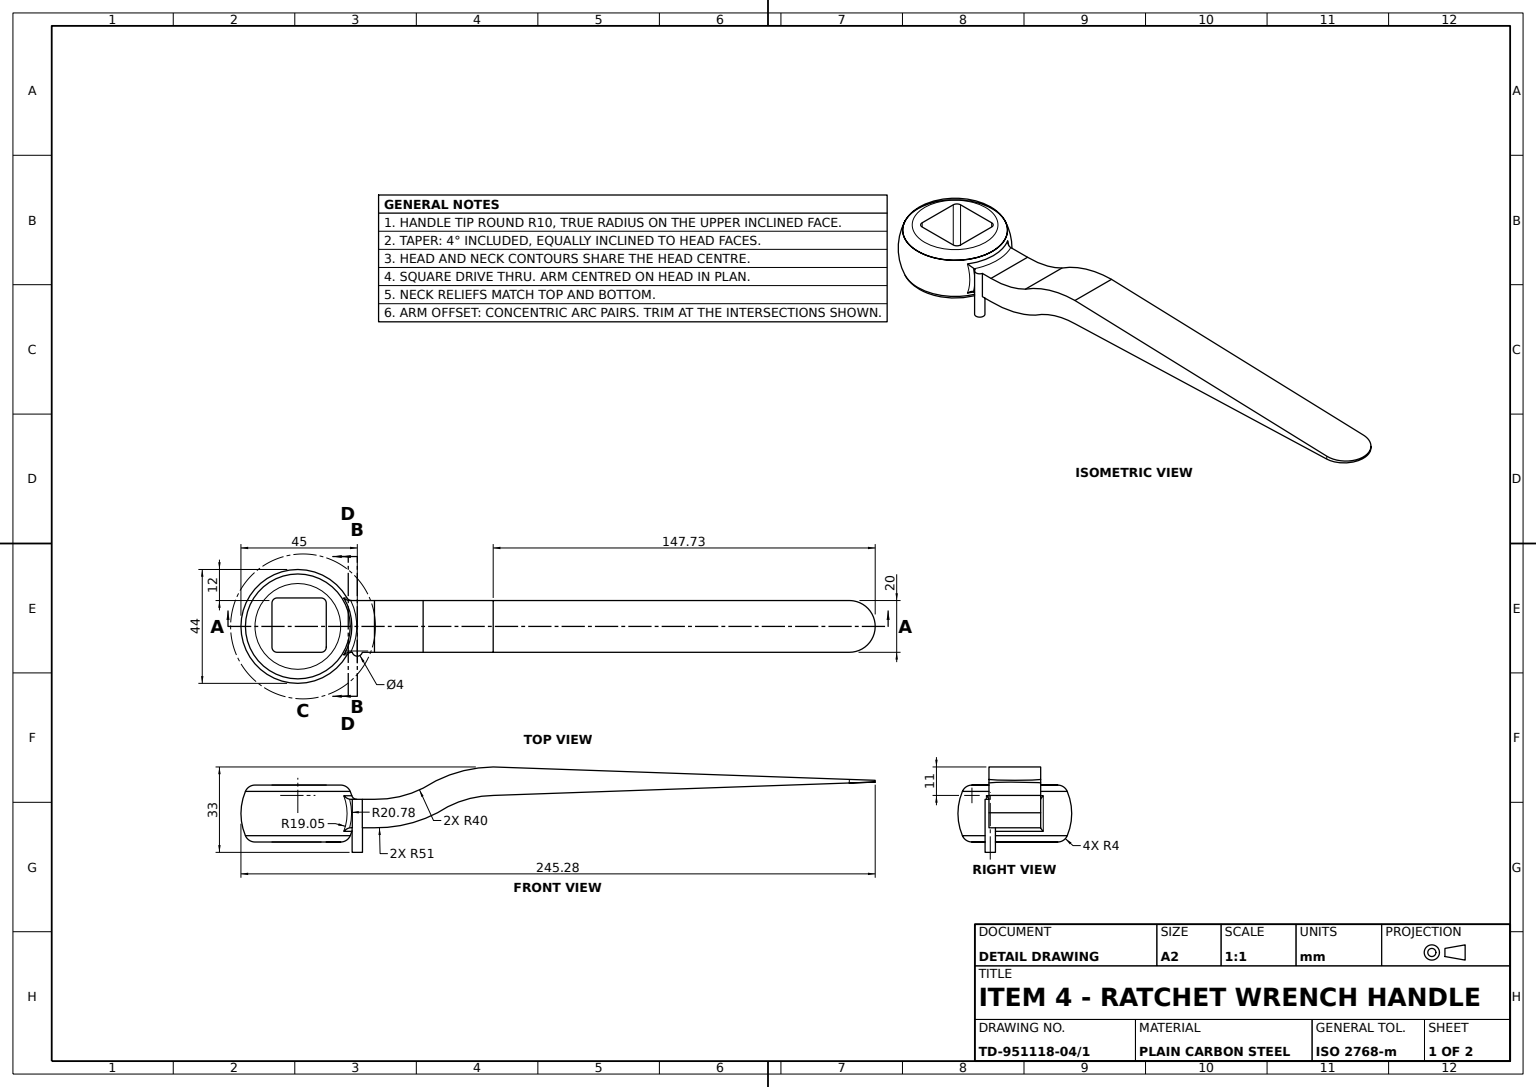
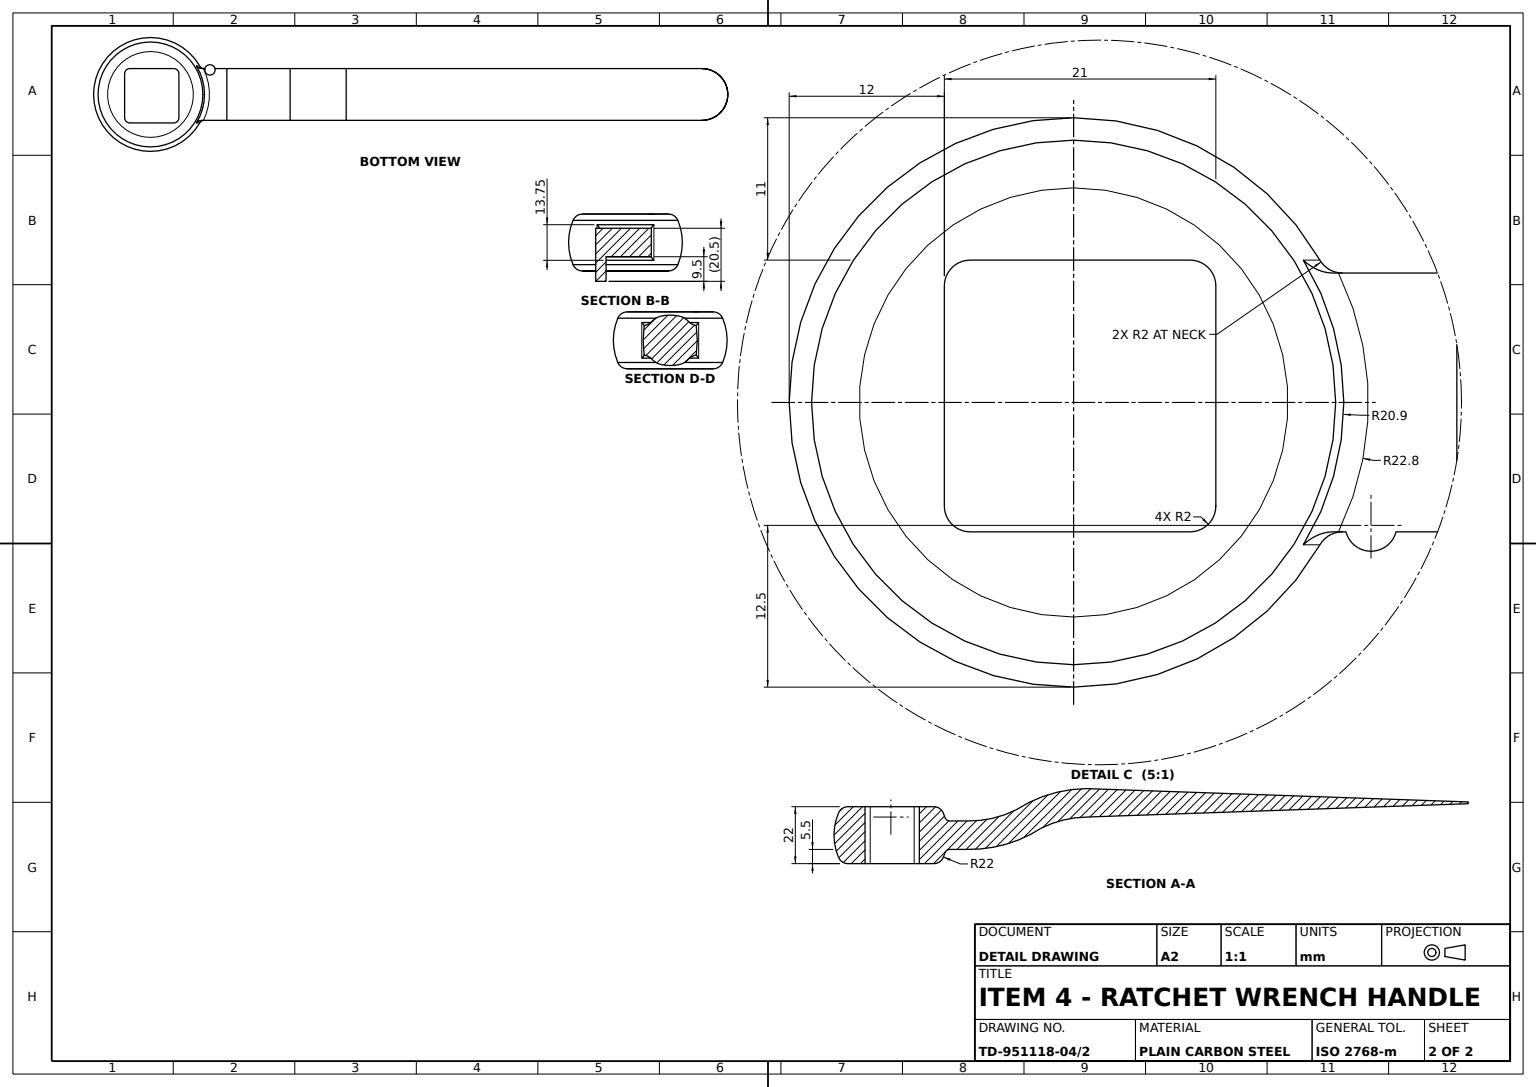
ISO-10303-21;
HEADER;
FILE_DESCRIPTION((''),'2;1');
FILE_NAME('','',(''),(''),'','','');
FILE_SCHEMA(('AUTOMOTIVE_DESIGN'));
ENDSEC;
DATA;
#1=APPLICATION_CONTEXT('');
#2=PRODUCT_CONTEXT('',#1,'mechanical');
#3=PRODUCT('','','',(#2));
#4=PRODUCT_DEFINITION_FORMATION('','',#3);
#5=PRODUCT_DEFINITION_CONTEXT('',#1,'design');
#6=PRODUCT_DEFINITION('','',#4,#5);
#7=PRODUCT_DEFINITION_SHAPE('','',#6);
#8=(LENGTH_UNIT()NAMED_UNIT(*)SI_UNIT(.MILLI.,.METRE.));
#9=(NAMED_UNIT(*)PLANE_ANGLE_UNIT()SI_UNIT($,.RADIAN.));
#10=(NAMED_UNIT(*)SI_UNIT($,.STERADIAN.)SOLID_ANGLE_UNIT());
#11=UNCERTAINTY_MEASURE_WITH_UNIT(LENGTH_MEASURE(1.E-05),#8,'distance_accuracy_value','');
#12=(GEOMETRIC_REPRESENTATION_CONTEXT(3)GLOBAL_UNCERTAINTY_ASSIGNED_CONTEXT((#11))GLOBAL_UNIT_ASSIGNED_CONTEXT((#8,#9,#10))REPRESENTATION_CONTEXT('',''));
#13=CARTESIAN_POINT('',(42.78461,0.,-10.));
#14=VERTEX_POINT('',#13);
#15=CARTESIAN_POINT('',(42.032076,5.542194,-10.));
#16=VERTEX_POINT('',#15);
#17=CARTESIAN_POINT('',(22.,0.,-10.));
#18=DIRECTION('',(0.,0.,1.));
#19=DIRECTION('',(1.,0.,0.));
#20=AXIS2_PLACEMENT_3D('',#17,#18,#19);
#21=CIRCLE('',#20,20.78461);
#22=EDGE_CURVE('',#14,#16,#21,.T.);
#23=ORIENTED_EDGE('',*,*,#22,.F.);
#24=CARTESIAN_POINT('',(41.052559,0.,-11.));
#25=VERTEX_POINT('',#24);
#26=CARTESIAN_POINT('',(42.78461,0.,-12.));
#27=DIRECTION('',(0.,-1.,0.));
#28=DIRECTION('',(0.,0.,-1.));
#29=AXIS2_PLACEMENT_3D('',#26,#27,#28);
#30=CIRCLE('',#29,2.);
#31=EDGE_CURVE('',#14,#25,#30,.T.);
#32=ORIENTED_EDGE('',*,*,#31,.T.);
#33=CARTESIAN_POINT('',(39.768916,6.875,-11.));
#34=VERTEX_POINT('',#33);
#35=CARTESIAN_POINT('',(22.,0.,-11.));
#36=AXIS2_PLACEMENT_3D('',#35,#28,#19);
#37=CIRCLE('',#36,19.052559);
#38=EDGE_CURVE('',#34,#25,#37,.T.);
#39=ORIENTED_EDGE('',*,*,#38,.F.);
#40=CARTESIAN_POINT('',(41.792387,5.586957,-10.));
#41=CARTESIAN_POINT('',(41.567371,5.660833,-10.034488));
#42=CARTESIAN_POINT('',(41.135793,5.845017,-10.14725));
#43=CARTESIAN_POINT('',(40.934143,5.954044,-10.225125));
#44=CARTESIAN_POINT('',(40.372609,6.307624,-10.497561));
#45=CARTESIAN_POINT('',(40.044195,6.58562,-10.736189));
#46=B_SPLINE_CURVE_WITH_KNOTS('',3,(#15,#40,#41,#42,#43,#44,#45,#33),.UNSPECIFIED.,.F.,.F.,(4,2,2,4),(0.,0.00071799,0.00143598,0.002871961),.UNSPECIFIED.);
#47=EDGE_CURVE('',#16,#34,#46,.T.);
#48=ORIENTED_EDGE('',*,*,#47,.F.);
#49=EDGE_LOOP('',(#23,#32,#39,#48));
#50=FACE_OUTER_BOUND('',#49,.T.);
#51=CARTESIAN_POINT('',(22.,0.,-12.));
#52=AXIS2_PLACEMENT_3D('',#51,#18,#19);
#53=TOROIDAL_SURFACE('',#52,20.78461,2.);
#54=ADVANCED_FACE('',(#50),#53,.F.);
#55=CARTESIAN_POINT('',(97.687925,7.000834,10.));
#56=VERTEX_POINT('',#55);
#57=CARTESIAN_POINT('',(235.240159,11.804263,10.));
#58=VERTEX_POINT('',#57);
#59=CARTESIAN_POINT('',(-0.125195,3.585124,10.));
#60=DIRECTION('',(0.999390827,0.034899497,0.));
#61=VECTOR('',#60,1000.);
#62=LINE('',#59,#61);
#63=EDGE_CURVE('',#56,#58,#62,.T.);
#64=ORIENTED_EDGE('',*,*,#63,.F.);
#65=CARTESIAN_POINT('',(97.687925,7.000834,-10.));
#66=VERTEX_POINT('',#65);
#67=VECTOR('',#28,1000.);
#68=LINE('',#55,#67);
#69=EDGE_CURVE('',#56,#66,#68,.T.);
#70=ORIENTED_EDGE('',*,*,#69,.T.);
#71=CARTESIAN_POINT('',(235.240159,11.804263,-10.));
#72=VERTEX_POINT('',#71);
#73=CARTESIAN_POINT('',(-0.125195,3.585124,-10.));
#74=LINE('',#73,#61);
#75=EDGE_CURVE('',#66,#72,#74,.T.);
#76=ORIENTED_EDGE('',*,*,#75,.T.);
#77=CARTESIAN_POINT('',(255.276783,12.503958,10.));
#78=CARTESIAN_POINT('',(255.276783,12.503958,-10.));
#79=(BOUNDED_CURVE()B_SPLINE_CURVE(3,(#57,#77,#78,#71),.UNSPECIFIED.,.F.,.F.)B_SPLINE_CURVE_WITH_KNOTS((4,4),(4.71238898,7.853981634),.UNSPECIFIED.)CURVE()GEOMETRIC_REPRESENTATION_ITEM()RATIONAL_B_SPLINE_CURVE((1.,0.333333333,0.333333333,1.))REPRESENTATION_ITEM(''));
#80=EDGE_CURVE('',#58,#72,#79,.T.);
#81=ORIENTED_EDGE('',*,*,#80,.F.);
#82=EDGE_LOOP('',(#64,#70,#76,#81));
#83=FACE_OUTER_BOUND('',#82,.T.);
#84=DIRECTION('',(-0.034899497,0.999390827,0.));
#85=DIRECTION('',(-0.999390827,-0.034899497,0.));
#86=AXIS2_PLACEMENT_3D('',#59,#84,#85);
#87=PLANE('',#86);
#88=ADVANCED_FACE('',(#83),#87,.F.);
#89=CARTESIAN_POINT('',(33.,11.,8.));
#90=VERTEX_POINT('',#89);
#91=CARTESIAN_POINT('',(33.,11.,-9.));
#92=VERTEX_POINT('',#91);
#93=CARTESIAN_POINT('',(33.,11.,0.));
#94=LINE('',#93,#67);
#95=EDGE_CURVE('',#90,#92,#94,.T.);
#96=ORIENTED_EDGE('',*,*,#95,.T.);
#97=CARTESIAN_POINT('',(33.,-11.,-9.));
#98=VERTEX_POINT('',#97);
#99=VECTOR('',#27,1000.);
#100=LINE('',#97,#99);
#101=EDGE_CURVE('',#92,#98,#100,.T.);
#102=ORIENTED_EDGE('',*,*,#101,.T.);
#103=CARTESIAN_POINT('',(33.,-11.,8.));
#104=VERTEX_POINT('',#103);
#105=CARTESIAN_POINT('',(33.,-11.,-30.));
#106=LINE('',#105,#67);
#107=EDGE_CURVE('',#104,#98,#106,.T.);
#108=ORIENTED_EDGE('',*,*,#107,.F.);
#109=DIRECTION('',(0.,1.,0.));
#110=VECTOR('',#109,1000.);
#111=LINE('',#89,#110);
#112=EDGE_CURVE('',#104,#90,#111,.T.);
#113=ORIENTED_EDGE('',*,*,#112,.T.);
#114=EDGE_LOOP('',(#96,#102,#108,#113));
#115=FACE_OUTER_BOUND('',#114,.T.);
#116=CARTESIAN_POINT('',(33.,-49.,0.));
#117=AXIS2_PLACEMENT_3D('',#116,#19,#28);
#118=PLANE('',#117);
#119=ADVANCED_FACE('',(#115),#118,.F.);
#120=CARTESIAN_POINT('',(12.,11.,-9.));
#121=VERTEX_POINT('',#120);
#122=CARTESIAN_POINT('',(14.,11.,-11.));
#123=VERTEX_POINT('',#122);
#124=CARTESIAN_POINT('',(14.,11.,-9.));
#125=AXIS2_PLACEMENT_3D('',#124,#27,#28);
#126=CIRCLE('',#125,2.);
#127=EDGE_CURVE('',#121,#123,#126,.T.);
#128=ORIENTED_EDGE('',*,*,#127,.F.);
#129=CARTESIAN_POINT('',(12.,-11.,-9.));
#130=VERTEX_POINT('',#129);
#131=LINE('',#120,#110);
#132=EDGE_CURVE('',#130,#121,#131,.T.);
#133=ORIENTED_EDGE('',*,*,#132,.F.);
#134=CARTESIAN_POINT('',(14.,-11.,-11.));
#135=VERTEX_POINT('',#134);
#136=CARTESIAN_POINT('',(14.,-11.,-9.));
#137=AXIS2_PLACEMENT_3D('',#136,#109,#18);
#138=CIRCLE('',#137,2.);
#139=EDGE_CURVE('',#135,#130,#138,.T.);
#140=ORIENTED_EDGE('',*,*,#139,.F.);
#141=LINE('',#134,#99);
#142=EDGE_CURVE('',#123,#135,#141,.T.);
#143=ORIENTED_EDGE('',*,*,#142,.F.);
#144=EDGE_LOOP('',(#128,#133,#140,#143));
#145=FACE_OUTER_BOUND('',#144,.T.);
#146=CARTESIAN_POINT('',(14.,-49.,-9.));
#147=AXIS2_PLACEMENT_3D('',#146,#27,#28);
#148=CYLINDRICAL_SURFACE('',#147,2.);
#149=ADVANCED_FACE('',(#145),#148,.F.);
#150=CARTESIAN_POINT('',(12.,11.,8.));
#151=VERTEX_POINT('',#150);
#152=CARTESIAN_POINT('',(12.,-11.,8.));
#153=VERTEX_POINT('',#152);
#154=LINE('',#152,#99);
#155=EDGE_CURVE('',#151,#153,#154,.T.);
#156=ORIENTED_EDGE('',*,*,#155,.F.);
#157=CARTESIAN_POINT('',(14.,11.,10.));
#158=VERTEX_POINT('',#157);
#159=CARTESIAN_POINT('',(14.,11.,8.));
#160=AXIS2_PLACEMENT_3D('',#159,#27,#28);
#161=CIRCLE('',#160,2.);
#162=EDGE_CURVE('',#158,#151,#161,.T.);
#163=ORIENTED_EDGE('',*,*,#162,.F.);
#164=CARTESIAN_POINT('',(14.,-11.,10.));
#165=VERTEX_POINT('',#164);
#166=LINE('',#157,#110);
#167=EDGE_CURVE('',#165,#158,#166,.T.);
#168=ORIENTED_EDGE('',*,*,#167,.F.);
#169=CARTESIAN_POINT('',(14.,-11.,8.));
#170=AXIS2_PLACEMENT_3D('',#169,#109,#18);
#171=CIRCLE('',#170,2.);
#172=EDGE_CURVE('',#153,#165,#171,.T.);
#173=ORIENTED_EDGE('',*,*,#172,.F.);
#174=EDGE_LOOP('',(#156,#163,#168,#173));
#175=FACE_OUTER_BOUND('',#174,.T.);
#176=CARTESIAN_POINT('',(14.,-49.,8.));
#177=AXIS2_PLACEMENT_3D('',#176,#27,#28);
#178=CYLINDRICAL_SURFACE('',#177,2.);
#179=ADVANCED_FACE('',(#175),#178,.F.);
#180=CARTESIAN_POINT('',(43.,-15.,9.5));
#181=VERTEX_POINT('',#180);
#182=CARTESIAN_POINT('',(47.,-15.,9.5));
#183=VERTEX_POINT('',#182);
#184=CARTESIAN_POINT('',(45.,-15.,9.5));
#185=DIRECTION('',(-1.,0.,0.));
#186=AXIS2_PLACEMENT_3D('',#184,#109,#185);
#187=CIRCLE('',#186,2.);
#188=EDGE_CURVE('',#181,#183,#187,.T.);
#189=ORIENTED_EDGE('',*,*,#188,.F.);
#190=EDGE_CURVE('',#183,#181,#187,.T.);
#191=ORIENTED_EDGE('',*,*,#190,.F.);
#192=EDGE_LOOP('',(#189,#191));
#193=FACE_OUTER_BOUND('',#192,.T.);
#194=PLANE('',#186);
#195=ADVANCED_FACE('',(#193),#194,.F.);
#196=CARTESIAN_POINT('',(22.,11.,16.583124));
#197=VERTEX_POINT('',#196);
#198=CARTESIAN_POINT('',(22.,8.555556,20.268263));
#199=VERTEX_POINT('',#198);
#200=CARTESIAN_POINT('',(22.,7.,16.583124));
#201=AXIS2_PLACEMENT_3D('',#200,#19,#28);
#202=CIRCLE('',#201,4.);
#203=EDGE_CURVE('',#197,#199,#202,.T.);
#204=ORIENTED_EDGE('',*,*,#203,.T.);
#205=CARTESIAN_POINT('',(42.268263,8.555556,0.));
#206=VERTEX_POINT('',#205);
#207=CARTESIAN_POINT('',(22.,8.555556,0.));
#208=AXIS2_PLACEMENT_3D('',#207,#27,#28);
#209=CIRCLE('',#208,20.268263);
#210=EDGE_CURVE('',#206,#199,#209,.T.);
#211=ORIENTED_EDGE('',*,*,#210,.F.);
#212=CARTESIAN_POINT('',(22.,8.555556,-20.268263));
#213=VERTEX_POINT('',#212);
#214=EDGE_CURVE('',#213,#206,#209,.T.);
#215=ORIENTED_EDGE('',*,*,#214,.F.);
#216=CARTESIAN_POINT('',(22.,11.,-16.583124));
#217=VERTEX_POINT('',#216);
#218=CARTESIAN_POINT('',(22.,7.,-16.583124));
#219=AXIS2_PLACEMENT_3D('',#218,#185,#18);
#220=CIRCLE('',#219,4.);
#221=EDGE_CURVE('',#217,#213,#220,.T.);
#222=ORIENTED_EDGE('',*,*,#221,.F.);
#223=CARTESIAN_POINT('',(22.,11.,0.));
#224=AXIS2_PLACEMENT_3D('',#223,#109,#28);
#225=CIRCLE('',#224,16.583124);
#226=EDGE_CURVE('',#197,#217,#225,.T.);
#227=ORIENTED_EDGE('',*,*,#226,.F.);
#228=EDGE_LOOP('',(#204,#211,#215,#222,#227));
#229=FACE_OUTER_BOUND('',#228,.T.);
#230=CARTESIAN_POINT('',(22.,7.,0.));
#231=AXIS2_PLACEMENT_3D('',#230,#27,#28);
#232=TOROIDAL_SURFACE('',#231,16.583124,4.);
#233=ADVANCED_FACE('',(#229),#232,.T.);
#234=CARTESIAN_POINT('',(12.,11.,-11.));
#235=VECTOR('',#18,1000.);
#236=LINE('',#234,#235);
#237=EDGE_CURVE('',#121,#151,#236,.T.);
#238=ORIENTED_EDGE('',*,*,#237,.T.);
#239=ORIENTED_EDGE('',*,*,#155,.T.);
#240=CARTESIAN_POINT('',(12.,-11.,-30.));
#241=LINE('',#240,#235);
#242=EDGE_CURVE('',#130,#153,#241,.T.);
#243=ORIENTED_EDGE('',*,*,#242,.F.);
#244=ORIENTED_EDGE('',*,*,#132,.T.);
#245=EDGE_LOOP('',(#238,#239,#243,#244));
#246=FACE_OUTER_BOUND('',#245,.T.);
#247=CARTESIAN_POINT('',(12.,-49.,-11.));
#248=AXIS2_PLACEMENT_3D('',#247,#185,#18);
#249=PLANE('',#248);
#250=ADVANCED_FACE('',(#246),#249,.F.);
#251=CARTESIAN_POINT('',(70.459551,9.812249,10.));
#252=VERTEX_POINT('',#251);
#253=CARTESIAN_POINT('',(70.459551,9.812249,-10.));
#254=VERTEX_POINT('',#253);
#255=LINE('',#251,#67);
#256=EDGE_CURVE('',#252,#254,#255,.T.);
#257=ORIENTED_EDGE('',*,*,#256,.F.);
#258=CARTESIAN_POINT('',(97.552511,18.,10.));
#259=VERTEX_POINT('',#258);
#260=CARTESIAN_POINT('',(98.180342,-32.996135,10.));
#261=AXIS2_PLACEMENT_3D('',#260,#28,#19);
#262=CIRCLE('',#261,51.);
#263=EDGE_CURVE('',#252,#259,#262,.T.);
#264=ORIENTED_EDGE('',*,*,#263,.T.);
#265=CARTESIAN_POINT('',(97.552511,18.,-10.));
#266=VERTEX_POINT('',#265);
#267=LINE('',#258,#67);
#268=EDGE_CURVE('',#259,#266,#267,.T.);
#269=ORIENTED_EDGE('',*,*,#268,.T.);
#270=CARTESIAN_POINT('',(98.180342,-32.996135,-10.));
#271=AXIS2_PLACEMENT_3D('',#270,#28,#19);
#272=CIRCLE('',#271,51.);
#273=EDGE_CURVE('',#254,#266,#272,.T.);
#274=ORIENTED_EDGE('',*,*,#273,.F.);
#275=EDGE_LOOP('',(#257,#264,#269,#274));
#276=FACE_OUTER_BOUND('',#275,.T.);
#277=AXIS2_PLACEMENT_3D('',#260,#28,#185);
#278=CYLINDRICAL_SURFACE('',#277,51.);
#279=ADVANCED_FACE('',(#276),#278,.T.);
#280=CARTESIAN_POINT('',(46.936492,-5.5,10.));
#281=VERTEX_POINT('',#280);
#282=CARTESIAN_POINT('',(51.544356,-5.5,10.));
#283=VERTEX_POINT('',#282);
#284=CARTESIAN_POINT('',(0.,-5.5,10.));
#285=VECTOR('',#19,1000.);
#286=LINE('',#284,#285);
#287=EDGE_CURVE('',#281,#283,#286,.T.);
#288=ORIENTED_EDGE('',*,*,#287,.T.);
#289=CARTESIAN_POINT('',(76.011119,0.298392,10.));
#290=VERTEX_POINT('',#289);
#291=CARTESIAN_POINT('',(52.379923,45.493155,10.));
#292=AXIS2_PLACEMENT_3D('',#291,#18,#19);
#293=CIRCLE('',#292,51.);
#294=EDGE_CURVE('',#283,#290,#293,.T.);
#295=ORIENTED_EDGE('',*,*,#294,.T.);
#296=CIRCLE('',#261,40.);
#297=EDGE_CURVE('',#290,#56,#296,.T.);
#298=ORIENTED_EDGE('',*,*,#297,.T.);
#299=ORIENTED_EDGE('',*,*,#63,.T.);
#300=CARTESIAN_POINT('',(235.288555,13.190151,10.));
#301=VERTEX_POINT('',#300);
#302=CARTESIAN_POINT('',(234.171771,-18.790355,10.));
#303=DIRECTION('',(0.034899497,0.999390827,0.));
#304=VECTOR('',#303,1000.);
#305=LINE('',#302,#304);
#306=EDGE_CURVE('',#58,#301,#305,.T.);
#307=ORIENTED_EDGE('',*,*,#306,.T.);
#308=CARTESIAN_POINT('',(0.746625,21.380536,10.));
#309=DIRECTION('',(0.999390827,-0.034899497,0.));
#310=VECTOR('',#309,1000.);
#311=LINE('',#308,#310);
#312=EDGE_CURVE('',#259,#301,#311,.T.);
#313=ORIENTED_EDGE('',*,*,#312,.F.);
#314=ORIENTED_EDGE('',*,*,#263,.F.);
#315=CARTESIAN_POINT('',(51.639939,5.5,10.));
#316=VERTEX_POINT('',#315);
#317=CIRCLE('',#292,40.);
#318=EDGE_CURVE('',#316,#252,#317,.T.);
#319=ORIENTED_EDGE('',*,*,#318,.F.);
#320=CARTESIAN_POINT('',(46.936492,5.5,10.));
#321=VERTEX_POINT('',#320);
#322=CARTESIAN_POINT('',(0.,5.5,10.));
#323=LINE('',#322,#285);
#324=EDGE_CURVE('',#321,#316,#323,.T.);
#325=ORIENTED_EDGE('',*,*,#324,.F.);
#326=CARTESIAN_POINT('',(46.936492,-15.,10.));
#327=LINE('',#326,#110);
#328=EDGE_CURVE('',#281,#321,#327,.T.);
#329=ORIENTED_EDGE('',*,*,#328,.F.);
#330=EDGE_LOOP('',(#288,#295,#298,#299,#307,#313,#314,#319,#325,#329));
#331=FACE_OUTER_BOUND('',#330,.T.);
#332=CARTESIAN_POINT('',(0.,0.,10.));
#333=AXIS2_PLACEMENT_3D('',#332,#18,#19);
#334=PLANE('',#333);
#335=ADVANCED_FACE('',(#331),#334,.T.);
#336=CARTESIAN_POINT('',(1.731737,-8.555556,0.));
#337=VERTEX_POINT('',#336);
#338=CARTESIAN_POINT('',(0.,0.,0.));
#339=VERTEX_POINT('',#338);
#340=CARTESIAN_POINT('',(22.,0.,0.));
#341=AXIS2_PLACEMENT_3D('',#340,#28,#109);
#342=CIRCLE('',#341,22.);
#343=EDGE_CURVE('',#337,#339,#342,.T.);
#344=ORIENTED_EDGE('',*,*,#343,.T.);
#345=CARTESIAN_POINT('',(1.731737,8.555556,0.));
#346=VERTEX_POINT('',#345);
#347=AXIS2_PLACEMENT_3D('',#340,#18,#19);
#348=CIRCLE('',#347,22.);
#349=EDGE_CURVE('',#346,#339,#348,.T.);
#350=ORIENTED_EDGE('',*,*,#349,.F.);
#351=EDGE_CURVE('',#346,#213,#209,.T.);
#352=ORIENTED_EDGE('',*,*,#351,.T.);
#353=ORIENTED_EDGE('',*,*,#214,.T.);
#354=CARTESIAN_POINT('',(42.898191,6.875,0.));
#355=VERTEX_POINT('',#354);
#356=EDGE_CURVE('',#355,#206,#348,.T.);
#357=ORIENTED_EDGE('',*,*,#356,.F.);
#358=CARTESIAN_POINT('',(22.,6.875,0.));
#359=AXIS2_PLACEMENT_3D('',#358,#109,#19);
#360=CIRCLE('',#359,20.898191);
#361=EDGE_CURVE('',#355,#34,#360,.T.);
#362=ORIENTED_EDGE('',*,*,#361,.T.);
#363=ORIENTED_EDGE('',*,*,#38,.T.);
#364=CARTESIAN_POINT('',(39.768916,-6.875,-11.));
#365=VERTEX_POINT('',#364);
#366=EDGE_CURVE('',#25,#365,#37,.T.);
#367=ORIENTED_EDGE('',*,*,#366,.T.);
#368=CARTESIAN_POINT('',(42.898191,-6.875,0.));
#369=VERTEX_POINT('',#368);
#370=CARTESIAN_POINT('',(22.,-6.875,0.));
#371=AXIS2_PLACEMENT_3D('',#370,#27,#18);
#372=CIRCLE('',#371,20.898191);
#373=EDGE_CURVE('',#365,#369,#372,.T.);
#374=ORIENTED_EDGE('',*,*,#373,.T.);
#375=CARTESIAN_POINT('',(42.268263,-8.555556,0.));
#376=VERTEX_POINT('',#375);
#377=EDGE_CURVE('',#369,#376,#342,.T.);
#378=ORIENTED_EDGE('',*,*,#377,.T.);
#379=CARTESIAN_POINT('',(22.,-8.555556,-20.268263));
#380=VERTEX_POINT('',#379);
#381=CARTESIAN_POINT('',(22.,-8.555556,0.));
#382=AXIS2_PLACEMENT_3D('',#381,#109,#18);
#383=CIRCLE('',#382,20.268263);
#384=EDGE_CURVE('',#376,#380,#383,.T.);
#385=ORIENTED_EDGE('',*,*,#384,.T.);
#386=EDGE_CURVE('',#380,#337,#383,.T.);
#387=ORIENTED_EDGE('',*,*,#386,.T.);
#388=EDGE_LOOP('',(#344,#350,#352,#353,#357,#362,#363,#367,#374,#378,#385,#387));
#389=FACE_OUTER_BOUND('',#388,.T.);
#390=SPHERICAL_SURFACE('',#341,22.);
#391=ADVANCED_FACE('',(#389),#390,.T.);
#392=CARTESIAN_POINT('',(42.487801,5.5,10.));
#393=VERTEX_POINT('',#392);
#394=CARTESIAN_POINT('',(43.063508,5.5,10.));
#395=VERTEX_POINT('',#394);
#396=EDGE_CURVE('',#393,#395,#323,.T.);
#397=ORIENTED_EDGE('',*,*,#396,.T.);
#398=CARTESIAN_POINT('',(45.,5.5,9.5));
#399=AXIS2_PLACEMENT_3D('',#398,#109,#185);
#400=CIRCLE('',#399,2.);
#401=EDGE_CURVE('',#395,#321,#400,.T.);
#402=ORIENTED_EDGE('',*,*,#401,.T.);
#403=ORIENTED_EDGE('',*,*,#324,.T.);
#404=CARTESIAN_POINT('',(51.639939,5.5,-10.));
#405=VERTEX_POINT('',#404);
#406=LINE('',#315,#67);
#407=EDGE_CURVE('',#316,#405,#406,.T.);
#408=ORIENTED_EDGE('',*,*,#407,.T.);
#409=CARTESIAN_POINT('',(42.487801,5.5,-10.));
#410=VERTEX_POINT('',#409);
#411=CARTESIAN_POINT('',(0.,5.5,-10.));
#412=LINE('',#411,#285);
#413=EDGE_CURVE('',#410,#405,#412,.T.);
#414=ORIENTED_EDGE('',*,*,#413,.F.);
#415=CARTESIAN_POINT('',(22.,5.5,0.));
#416=AXIS2_PLACEMENT_3D('',#415,#27,#185);
#417=CIRCLE('',#416,22.798026);
#418=EDGE_CURVE('',#410,#393,#417,.T.);
#419=ORIENTED_EDGE('',*,*,#418,.T.);
#420=EDGE_LOOP('',(#397,#402,#403,#408,#414,#419));
#421=FACE_OUTER_BOUND('',#420,.T.);
#422=AXIS2_PLACEMENT_3D('',#322,#109,#185);
#423=PLANE('',#422);
#424=ADVANCED_FACE('',(#421),#423,.T.);
#425=ORIENTED_EDGE('',*,*,#256,.T.);
#426=CARTESIAN_POINT('',(52.379923,45.493155,-10.));
#427=AXIS2_PLACEMENT_3D('',#426,#18,#19);
#428=CIRCLE('',#427,40.);
#429=EDGE_CURVE('',#405,#254,#428,.T.);
#430=ORIENTED_EDGE('',*,*,#429,.F.);
#431=ORIENTED_EDGE('',*,*,#407,.F.);
#432=ORIENTED_EDGE('',*,*,#318,.T.);
#433=EDGE_LOOP('',(#425,#430,#431,#432));
#434=FACE_OUTER_BOUND('',#433,.T.);
#435=AXIS2_PLACEMENT_3D('',#291,#28,#185);
#436=CYLINDRICAL_SURFACE('',#435,40.);
#437=ADVANCED_FACE('',(#434),#436,.F.);
#438=ORIENTED_EDGE('',*,*,#297,.F.);
#439=CARTESIAN_POINT('',(76.011119,0.298392,-10.));
#440=VERTEX_POINT('',#439);
#441=LINE('',#289,#67);
#442=EDGE_CURVE('',#290,#440,#441,.T.);
#443=ORIENTED_EDGE('',*,*,#442,.T.);
#444=CIRCLE('',#271,40.);
#445=EDGE_CURVE('',#440,#66,#444,.T.);
#446=ORIENTED_EDGE('',*,*,#445,.T.);
#447=ORIENTED_EDGE('',*,*,#69,.F.);
#448=EDGE_LOOP('',(#438,#443,#446,#447));
#449=FACE_OUTER_BOUND('',#448,.T.);
#450=CYLINDRICAL_SURFACE('',#277,40.);
#451=ADVANCED_FACE('',(#449),#450,.F.);
#452=CARTESIAN_POINT('',(31.,11.,-11.));
#453=VERTEX_POINT('',#452);
#454=CARTESIAN_POINT('',(31.,11.,-9.));
#455=AXIS2_PLACEMENT_3D('',#454,#27,#28);
#456=CIRCLE('',#455,2.);
#457=EDGE_CURVE('',#453,#92,#456,.T.);
#458=ORIENTED_EDGE('',*,*,#457,.F.);
#459=CARTESIAN_POINT('',(31.,-11.,-11.));
#460=VERTEX_POINT('',#459);
#461=LINE('',#452,#110);
#462=EDGE_CURVE('',#460,#453,#461,.T.);
#463=ORIENTED_EDGE('',*,*,#462,.F.);
#464=CARTESIAN_POINT('',(31.,-11.,-9.));
#465=AXIS2_PLACEMENT_3D('',#464,#109,#18);
#466=CIRCLE('',#465,2.);
#467=EDGE_CURVE('',#98,#460,#466,.T.);
#468=ORIENTED_EDGE('',*,*,#467,.F.);
#469=ORIENTED_EDGE('',*,*,#101,.F.);
#470=EDGE_LOOP('',(#458,#463,#468,#469));
#471=FACE_OUTER_BOUND('',#470,.T.);
#472=CARTESIAN_POINT('',(31.,-49.,-9.));
#473=AXIS2_PLACEMENT_3D('',#472,#27,#28);
#474=CYLINDRICAL_SURFACE('',#473,2.);
#475=ADVANCED_FACE('',(#471),#474,.F.);
#476=CARTESIAN_POINT('',(31.,-11.,10.));
#477=VERTEX_POINT('',#476);
#478=CARTESIAN_POINT('',(31.,-11.,8.));
#479=AXIS2_PLACEMENT_3D('',#478,#109,#18);
#480=CIRCLE('',#479,2.);
#481=EDGE_CURVE('',#477,#104,#480,.T.);
#482=ORIENTED_EDGE('',*,*,#481,.F.);
#483=CARTESIAN_POINT('',(31.,11.,10.));
#484=VERTEX_POINT('',#483);
#485=LINE('',#476,#99);
#486=EDGE_CURVE('',#484,#477,#485,.T.);
#487=ORIENTED_EDGE('',*,*,#486,.F.);
#488=CARTESIAN_POINT('',(31.,11.,8.));
#489=AXIS2_PLACEMENT_3D('',#488,#27,#28);
#490=CIRCLE('',#489,2.);
#491=EDGE_CURVE('',#90,#484,#490,.T.);
#492=ORIENTED_EDGE('',*,*,#491,.F.);
#493=ORIENTED_EDGE('',*,*,#112,.F.);
#494=EDGE_LOOP('',(#482,#487,#492,#493));
#495=FACE_OUTER_BOUND('',#494,.T.);
#496=CARTESIAN_POINT('',(31.,-49.,8.));
#497=AXIS2_PLACEMENT_3D('',#496,#27,#28);
#498=CYLINDRICAL_SURFACE('',#497,2.);
#499=ADVANCED_FACE('',(#495),#498,.F.);
#500=CARTESIAN_POINT('',(42.032076,5.542194,10.));
#501=VERTEX_POINT('',#500);
#502=CARTESIAN_POINT('',(39.768916,6.875,11.));
#503=VERTEX_POINT('',#502);
#504=CARTESIAN_POINT('',(41.792387,5.586957,10.));
#505=CARTESIAN_POINT('',(41.567371,5.660833,10.034488));
#506=CARTESIAN_POINT('',(41.135793,5.845017,10.14725));
#507=CARTESIAN_POINT('',(40.934143,5.954044,10.225125));
#508=CARTESIAN_POINT('',(40.372609,6.307624,10.497561));
#509=CARTESIAN_POINT('',(40.044195,6.58562,10.736189));
#510=B_SPLINE_CURVE_WITH_KNOTS('',3,(#500,#504,#505,#506,#507,#508,#509,#502),.UNSPECIFIED.,.F.,.F.,(4,2,2,4),(0.,0.00071799,0.00143598,0.002871961),.UNSPECIFIED.);
#511=EDGE_CURVE('',#501,#503,#510,.T.);
#512=ORIENTED_EDGE('',*,*,#511,.T.);
#513=CARTESIAN_POINT('',(41.052559,0.,11.));
#514=VERTEX_POINT('',#513);
#515=CARTESIAN_POINT('',(22.,0.,11.));
#516=AXIS2_PLACEMENT_3D('',#515,#18,#185);
#517=CIRCLE('',#516,19.052559);
#518=EDGE_CURVE('',#514,#503,#517,.T.);
#519=ORIENTED_EDGE('',*,*,#518,.F.);
#520=CARTESIAN_POINT('',(42.78461,0.,10.));
#521=VERTEX_POINT('',#520);
#522=CARTESIAN_POINT('',(42.78461,0.,12.));
#523=AXIS2_PLACEMENT_3D('',#522,#27,#28);
#524=CIRCLE('',#523,2.);
#525=EDGE_CURVE('',#514,#521,#524,.T.);
#526=ORIENTED_EDGE('',*,*,#525,.T.);
#527=CARTESIAN_POINT('',(22.,0.,10.));
#528=AXIS2_PLACEMENT_3D('',#527,#28,#19);
#529=CIRCLE('',#528,20.78461);
#530=EDGE_CURVE('',#501,#521,#529,.T.);
#531=ORIENTED_EDGE('',*,*,#530,.F.);
#532=EDGE_LOOP('',(#512,#519,#526,#531));
#533=FACE_OUTER_BOUND('',#532,.T.);
#534=CARTESIAN_POINT('',(22.,0.,12.));
#535=AXIS2_PLACEMENT_3D('',#534,#18,#19);
#536=TOROIDAL_SURFACE('',#535,20.78461,2.);
#537=ADVANCED_FACE('',(#533),#536,.F.);
#538=ORIENTED_EDGE('',*,*,#445,.F.);
#539=CARTESIAN_POINT('',(51.544356,-5.5,-10.));
#540=VERTEX_POINT('',#539);
#541=CIRCLE('',#427,51.);
#542=EDGE_CURVE('',#540,#440,#541,.T.);
#543=ORIENTED_EDGE('',*,*,#542,.F.);
#544=CARTESIAN_POINT('',(42.487801,-5.5,-10.));
#545=VERTEX_POINT('',#544);
#546=CARTESIAN_POINT('',(0.,-5.5,-10.));
#547=LINE('',#546,#285);
#548=EDGE_CURVE('',#545,#540,#547,.T.);
#549=ORIENTED_EDGE('',*,*,#548,.F.);
#550=CARTESIAN_POINT('',(42.032076,-5.542194,-10.));
#551=VERTEX_POINT('',#550);
#552=CARTESIAN_POINT('',(42.333516,-5.5,-10.));
#553=CARTESIAN_POINT('',(42.181642,-5.514262,-10.));
#554=B_SPLINE_CURVE_WITH_KNOTS('',3,(#544,#552,#553,#550),.UNSPECIFIED.,.F.,.F.,(4,4),(0.,0.000456385),.UNSPECIFIED.);
#555=EDGE_CURVE('',#545,#551,#554,.T.);
#556=ORIENTED_EDGE('',*,*,#555,.T.);
#557=EDGE_CURVE('',#551,#14,#21,.T.);
#558=ORIENTED_EDGE('',*,*,#557,.T.);
#559=ORIENTED_EDGE('',*,*,#22,.T.);
#560=CARTESIAN_POINT('',(42.182235,5.514152,-10.));
#561=CARTESIAN_POINT('',(42.334132,5.5,-10.));
#562=B_SPLINE_CURVE_WITH_KNOTS('',3,(#15,#560,#561,#409),.UNSPECIFIED.,.F.,.F.,(4,4),(0.002228682,0.002683644),.UNSPECIFIED.);
#563=EDGE_CURVE('',#16,#410,#562,.T.);
#564=ORIENTED_EDGE('',*,*,#563,.T.);
#565=ORIENTED_EDGE('',*,*,#413,.T.);
#566=ORIENTED_EDGE('',*,*,#429,.T.);
#567=ORIENTED_EDGE('',*,*,#273,.T.);
#568=CARTESIAN_POINT('',(235.288555,13.190151,-10.));
#569=VERTEX_POINT('',#568);
#570=CARTESIAN_POINT('',(0.746625,21.380536,-10.));
#571=LINE('',#570,#310);
#572=EDGE_CURVE('',#266,#569,#571,.T.);
#573=ORIENTED_EDGE('',*,*,#572,.T.);
#574=CARTESIAN_POINT('',(234.171771,-18.790355,-10.));
#575=LINE('',#574,#304);
#576=EDGE_CURVE('',#72,#569,#575,.T.);
#577=ORIENTED_EDGE('',*,*,#576,.F.);
#578=ORIENTED_EDGE('',*,*,#75,.F.);
#579=EDGE_LOOP('',(#538,#543,#549,#556,#558,#559,#564,#565,#566,#567,#573,#577,#578));
#580=FACE_OUTER_BOUND('',#579,.T.);
#581=CARTESIAN_POINT('',(0.,0.,-10.));
#582=AXIS2_PLACEMENT_3D('',#581,#18,#19);
#583=PLANE('',#582);
#584=ADVANCED_FACE('',(#580),#583,.F.);
#585=ORIENTED_EDGE('',*,*,#356,.T.);
#586=ORIENTED_EDGE('',*,*,#210,.T.);
#587=EDGE_CURVE('',#199,#346,#209,.T.);
#588=ORIENTED_EDGE('',*,*,#587,.T.);
#589=ORIENTED_EDGE('',*,*,#349,.T.);
#590=ORIENTED_EDGE('',*,*,#343,.F.);
#591=CARTESIAN_POINT('',(22.,-8.555556,20.268263));
#592=VERTEX_POINT('',#591);
#593=EDGE_CURVE('',#337,#592,#383,.T.);
#594=ORIENTED_EDGE('',*,*,#593,.T.);
#595=EDGE_CURVE('',#592,#376,#383,.T.);
#596=ORIENTED_EDGE('',*,*,#595,.T.);
#597=ORIENTED_EDGE('',*,*,#377,.F.);
#598=CARTESIAN_POINT('',(39.768916,-6.875,11.));
#599=VERTEX_POINT('',#598);
#600=EDGE_CURVE('',#369,#599,#372,.T.);
#601=ORIENTED_EDGE('',*,*,#600,.T.);
#602=EDGE_CURVE('',#599,#514,#517,.T.);
#603=ORIENTED_EDGE('',*,*,#602,.T.);
#604=ORIENTED_EDGE('',*,*,#518,.T.);
#605=EDGE_CURVE('',#503,#355,#360,.T.);
#606=ORIENTED_EDGE('',*,*,#605,.T.);
#607=EDGE_LOOP('',(#585,#586,#588,#589,#590,#594,#596,#597,#601,#603,#604,#606));
#608=FACE_OUTER_BOUND('',#607,.T.);
#609=ADVANCED_FACE('',(#608),#390,.T.);
#610=ORIENTED_EDGE('',*,*,#142,.T.);
#611=CARTESIAN_POINT('',(0.,-11.,-11.));
#612=VECTOR('',#185,1000.);
#613=LINE('',#611,#612);
#614=EDGE_CURVE('',#460,#135,#613,.T.);
#615=ORIENTED_EDGE('',*,*,#614,.F.);
#616=ORIENTED_EDGE('',*,*,#462,.T.);
#617=CARTESIAN_POINT('',(33.,11.,-11.));
#618=LINE('',#617,#612);
#619=EDGE_CURVE('',#453,#123,#618,.T.);
#620=ORIENTED_EDGE('',*,*,#619,.T.);
#621=EDGE_LOOP('',(#610,#615,#616,#620));
#622=FACE_OUTER_BOUND('',#621,.T.);
#623=CARTESIAN_POINT('',(33.,-49.,-11.));
#624=AXIS2_PLACEMENT_3D('',#623,#28,#185);
#625=PLANE('',#624);
#626=ADVANCED_FACE('',(#622),#625,.F.);
#627=CARTESIAN_POINT('',(43.,-5.5,9.5));
#628=VERTEX_POINT('',#627);
#629=CARTESIAN_POINT('',(43.063508,-5.5,10.));
#630=VERTEX_POINT('',#629);
#631=CARTESIAN_POINT('',(45.,-5.5,9.5));
#632=AXIS2_PLACEMENT_3D('',#631,#109,#18);
#633=CIRCLE('',#632,2.);
#634=EDGE_CURVE('',#628,#630,#633,.T.);
#635=ORIENTED_EDGE('',*,*,#634,.T.);
#636=CARTESIAN_POINT('',(42.487801,-5.5,10.));
#637=VERTEX_POINT('',#636);
#638=EDGE_CURVE('',#637,#630,#286,.T.);
#639=ORIENTED_EDGE('',*,*,#638,.F.);
#640=CARTESIAN_POINT('',(22.,-5.5,0.));
#641=AXIS2_PLACEMENT_3D('',#640,#109,#18);
#642=CIRCLE('',#641,22.798026);
#643=EDGE_CURVE('',#637,#545,#642,.T.);
#644=ORIENTED_EDGE('',*,*,#643,.T.);
#645=ORIENTED_EDGE('',*,*,#548,.T.);
#646=LINE('',#282,#67);
#647=EDGE_CURVE('',#283,#540,#646,.T.);
#648=ORIENTED_EDGE('',*,*,#647,.F.);
#649=ORIENTED_EDGE('',*,*,#287,.F.);
#650=CARTESIAN_POINT('',(47.,-5.5,9.5));
#651=VERTEX_POINT('',#650);
#652=EDGE_CURVE('',#281,#651,#633,.T.);
#653=ORIENTED_EDGE('',*,*,#652,.T.);
#654=EDGE_CURVE('',#651,#628,#633,.T.);
#655=ORIENTED_EDGE('',*,*,#654,.T.);
#656=EDGE_LOOP('',(#635,#639,#644,#645,#648,#649,#653,#655));
#657=FACE_OUTER_BOUND('',#656,.T.);
#658=AXIS2_PLACEMENT_3D('',#284,#109,#18);
#659=PLANE('',#658);
#660=ADVANCED_FACE('',(#657),#659,.F.);
#661=ORIENTED_EDGE('',*,*,#593,.F.);
#662=ORIENTED_EDGE('',*,*,#386,.F.);
#663=CARTESIAN_POINT('',(22.,-11.,-16.583124));
#664=VERTEX_POINT('',#663);
#665=CARTESIAN_POINT('',(22.,-7.,-16.583124));
#666=AXIS2_PLACEMENT_3D('',#665,#19,#28);
#667=CIRCLE('',#666,4.);
#668=EDGE_CURVE('',#664,#380,#667,.T.);
#669=ORIENTED_EDGE('',*,*,#668,.F.);
#670=CARTESIAN_POINT('',(22.,-11.,16.583124));
#671=VERTEX_POINT('',#670);
#672=CARTESIAN_POINT('',(22.,-11.,0.));
#673=AXIS2_PLACEMENT_3D('',#672,#27,#18);
#674=CIRCLE('',#673,16.583124);
#675=EDGE_CURVE('',#671,#664,#674,.T.);
#676=ORIENTED_EDGE('',*,*,#675,.F.);
#677=CARTESIAN_POINT('',(22.,-7.,16.583124));
#678=AXIS2_PLACEMENT_3D('',#677,#185,#18);
#679=CIRCLE('',#678,4.);
#680=EDGE_CURVE('',#671,#592,#679,.T.);
#681=ORIENTED_EDGE('',*,*,#680,.T.);
#682=EDGE_LOOP('',(#661,#662,#669,#676,#681));
#683=FACE_OUTER_BOUND('',#682,.T.);
#684=CARTESIAN_POINT('',(22.,-7.,0.));
#685=AXIS2_PLACEMENT_3D('',#684,#109,#18);
#686=TOROIDAL_SURFACE('',#685,16.583124,4.);
#687=ADVANCED_FACE('',(#683),#686,.T.);
#688=ORIENTED_EDGE('',*,*,#481,.T.);
#689=ORIENTED_EDGE('',*,*,#107,.T.);
#690=ORIENTED_EDGE('',*,*,#467,.T.);
#691=ORIENTED_EDGE('',*,*,#614,.T.);
#692=ORIENTED_EDGE('',*,*,#139,.T.);
#693=ORIENTED_EDGE('',*,*,#242,.T.);
#694=ORIENTED_EDGE('',*,*,#172,.T.);
#695=CARTESIAN_POINT('',(0.,-11.,10.));
#696=LINE('',#695,#285);
#697=EDGE_CURVE('',#165,#477,#696,.T.);
#698=ORIENTED_EDGE('',*,*,#697,.T.);
#699=EDGE_LOOP('',(#688,#689,#690,#691,#692,#693,#694,#698));
#700=FACE_BOUND('',#699,.T.);
#701=ORIENTED_EDGE('',*,*,#675,.T.);
#702=EDGE_CURVE('',#664,#671,#674,.T.);
#703=ORIENTED_EDGE('',*,*,#702,.T.);
#704=EDGE_LOOP('',(#701,#703));
#705=FACE_OUTER_BOUND('',#704,.T.);
#706=CARTESIAN_POINT('',(0.,-11.,-30.));
#707=AXIS2_PLACEMENT_3D('',#706,#109,#18);
#708=PLANE('',#707);
#709=ADVANCED_FACE('',(#700,#705),#708,.F.);
#710=ORIENTED_EDGE('',*,*,#294,.F.);
#711=ORIENTED_EDGE('',*,*,#647,.T.);
#712=ORIENTED_EDGE('',*,*,#542,.T.);
#713=ORIENTED_EDGE('',*,*,#442,.F.);
#714=EDGE_LOOP('',(#710,#711,#712,#713));
#715=FACE_OUTER_BOUND('',#714,.T.);
#716=CYLINDRICAL_SURFACE('',#435,51.);
#717=ADVANCED_FACE('',(#715),#716,.T.);
#718=ORIENTED_EDGE('',*,*,#668,.T.);
#719=ORIENTED_EDGE('',*,*,#384,.F.);
#720=ORIENTED_EDGE('',*,*,#595,.F.);
#721=ORIENTED_EDGE('',*,*,#680,.F.);
#722=ORIENTED_EDGE('',*,*,#702,.F.);
#723=EDGE_LOOP('',(#718,#719,#720,#721,#722));
#724=FACE_OUTER_BOUND('',#723,.T.);
#725=ADVANCED_FACE('',(#724),#686,.T.);
#726=CARTESIAN_POINT('',(40.045858,-6.583872,-10.734595));
#727=CARTESIAN_POINT('',(40.372634,-6.307606,-10.497545));
#728=CARTESIAN_POINT('',(40.934161,-5.954034,-10.225118));
#729=CARTESIAN_POINT('',(41.135808,-5.84501,-10.147245));
#730=CARTESIAN_POINT('',(41.567379,-5.66083,-10.034487));
#731=CARTESIAN_POINT('',(41.792392,-5.586956,-10.));
#732=B_SPLINE_CURVE_WITH_KNOTS('',3,(#364,#726,#727,#728,#729,#730,#731,#550),.UNSPECIFIED.,.F.,.F.,(4,2,2,4),(-0.000008643,0.001436013,0.002158341,0.002880669),.UNSPECIFIED.);
#733=EDGE_CURVE('',#365,#551,#732,.T.);
#734=ORIENTED_EDGE('',*,*,#733,.F.);
#735=ORIENTED_EDGE('',*,*,#366,.F.);
#736=ORIENTED_EDGE('',*,*,#31,.F.);
#737=ORIENTED_EDGE('',*,*,#557,.F.);
#738=EDGE_LOOP('',(#734,#735,#736,#737));
#739=FACE_OUTER_BOUND('',#738,.T.);
#740=ADVANCED_FACE('',(#739),#53,.F.);
#741=ORIENTED_EDGE('',*,*,#401,.F.);
#742=CARTESIAN_POINT('',(43.063508,-15.,10.));
#743=LINE('',#742,#99);
#744=EDGE_CURVE('',#395,#630,#743,.T.);
#745=ORIENTED_EDGE('',*,*,#744,.T.);
#746=ORIENTED_EDGE('',*,*,#634,.F.);
#747=LINE('',#180,#110);
#748=EDGE_CURVE('',#181,#628,#747,.T.);
#749=ORIENTED_EDGE('',*,*,#748,.F.);
#750=ORIENTED_EDGE('',*,*,#188,.T.);
#751=LINE('',#182,#110);
#752=EDGE_CURVE('',#183,#651,#751,.T.);
#753=ORIENTED_EDGE('',*,*,#752,.T.);
#754=ORIENTED_EDGE('',*,*,#652,.F.);
#755=ORIENTED_EDGE('',*,*,#328,.T.);
#756=EDGE_LOOP('',(#741,#745,#746,#749,#750,#753,#754,#755));
#757=FACE_OUTER_BOUND('',#756,.T.);
#758=CYLINDRICAL_SURFACE('',#186,2.);
#759=ADVANCED_FACE('',(#757),#758,.T.);
#760=ORIENTED_EDGE('',*,*,#643,.F.);
#761=CARTESIAN_POINT('',(42.032076,-5.542194,10.));
#762=VERTEX_POINT('',#761);
#763=CARTESIAN_POINT('',(42.182683,-5.514068,10.));
#764=CARTESIAN_POINT('',(42.334591,-5.5,10.));
#765=B_SPLINE_CURVE_WITH_KNOTS('',3,(#761,#763,#764,#636),.UNSPECIFIED.,.F.,.F.,(4,4),(0.,0.000457674),.UNSPECIFIED.);
#766=EDGE_CURVE('',#762,#637,#765,.T.);
#767=ORIENTED_EDGE('',*,*,#766,.F.);
#768=CARTESIAN_POINT('',(40.045858,-6.583872,10.734595));
#769=CARTESIAN_POINT('',(40.372634,-6.307606,10.497545));
#770=CARTESIAN_POINT('',(40.934161,-5.954034,10.225118));
#771=CARTESIAN_POINT('',(41.135808,-5.84501,10.147245));
#772=CARTESIAN_POINT('',(41.567379,-5.66083,10.034487));
#773=CARTESIAN_POINT('',(41.792392,-5.586956,10.));
#774=B_SPLINE_CURVE_WITH_KNOTS('',3,(#598,#768,#769,#770,#771,#772,#773,#761),.UNSPECIFIED.,.F.,.F.,(4,2,2,4),(-0.000008643,0.001436013,0.002158341,0.002880669),.UNSPECIFIED.);
#775=EDGE_CURVE('',#599,#762,#774,.T.);
#776=ORIENTED_EDGE('',*,*,#775,.F.);
#777=ORIENTED_EDGE('',*,*,#600,.F.);
#778=ORIENTED_EDGE('',*,*,#373,.F.);
#779=ORIENTED_EDGE('',*,*,#733,.T.);
#780=ORIENTED_EDGE('',*,*,#555,.F.);
#781=EDGE_LOOP('',(#760,#767,#776,#777,#778,#779,#780));
#782=FACE_OUTER_BOUND('',#781,.T.);
#783=CARTESIAN_POINT('',(22.,-7.5,0.));
#784=AXIS2_PLACEMENT_3D('',#783,#109,#18);
#785=TOROIDAL_SURFACE('',#784,22.798026,2.);
#786=ADVANCED_FACE('',(#782),#785,.F.);
#787=CARTESIAN_POINT('',(42.334591,5.5,10.));
#788=CARTESIAN_POINT('',(42.182683,5.514068,10.));
#789=B_SPLINE_CURVE_WITH_KNOTS('',3,(#392,#787,#788,#500),.UNSPECIFIED.,.F.,.F.,(4,4),(0.,0.000457674),.UNSPECIFIED.);
#790=EDGE_CURVE('',#393,#501,#789,.T.);
#791=ORIENTED_EDGE('',*,*,#790,.T.);
#792=ORIENTED_EDGE('',*,*,#530,.T.);
#793=EDGE_CURVE('',#521,#762,#529,.T.);
#794=ORIENTED_EDGE('',*,*,#793,.T.);
#795=ORIENTED_EDGE('',*,*,#766,.T.);
#796=ORIENTED_EDGE('',*,*,#638,.T.);
#797=ORIENTED_EDGE('',*,*,#744,.F.);
#798=ORIENTED_EDGE('',*,*,#396,.F.);
#799=EDGE_LOOP('',(#791,#792,#794,#795,#796,#797,#798));
#800=FACE_OUTER_BOUND('',#799,.T.);
#801=ADVANCED_FACE('',(#800),#334,.T.);
#802=ORIENTED_EDGE('',*,*,#602,.F.);
#803=ORIENTED_EDGE('',*,*,#775,.T.);
#804=ORIENTED_EDGE('',*,*,#793,.F.);
#805=ORIENTED_EDGE('',*,*,#525,.F.);
#806=EDGE_LOOP('',(#802,#803,#804,#805));
#807=FACE_OUTER_BOUND('',#806,.T.);
#808=ADVANCED_FACE('',(#807),#536,.F.);
#809=ORIENTED_EDGE('',*,*,#486,.T.);
#810=ORIENTED_EDGE('',*,*,#697,.F.);
#811=ORIENTED_EDGE('',*,*,#167,.T.);
#812=CARTESIAN_POINT('',(12.,11.,10.));
#813=LINE('',#812,#285);
#814=EDGE_CURVE('',#158,#484,#813,.T.);
#815=ORIENTED_EDGE('',*,*,#814,.T.);
#816=EDGE_LOOP('',(#809,#810,#811,#815));
#817=FACE_OUTER_BOUND('',#816,.T.);
#818=CARTESIAN_POINT('',(12.,-49.,10.));
#819=AXIS2_PLACEMENT_3D('',#818,#18,#19);
#820=PLANE('',#819);
#821=ADVANCED_FACE('',(#817),#820,.F.);
#822=ORIENTED_EDGE('',*,*,#563,.F.);
#823=ORIENTED_EDGE('',*,*,#47,.T.);
#824=ORIENTED_EDGE('',*,*,#361,.F.);
#825=ORIENTED_EDGE('',*,*,#605,.F.);
#826=ORIENTED_EDGE('',*,*,#511,.F.);
#827=ORIENTED_EDGE('',*,*,#790,.F.);
#828=ORIENTED_EDGE('',*,*,#418,.F.);
#829=EDGE_LOOP('',(#822,#823,#824,#825,#826,#827,#828));
#830=FACE_OUTER_BOUND('',#829,.T.);
#831=CARTESIAN_POINT('',(22.,7.5,0.));
#832=AXIS2_PLACEMENT_3D('',#831,#109,#185);
#833=TOROIDAL_SURFACE('',#832,22.798026,2.);
#834=ADVANCED_FACE('',(#830),#833,.F.);
#835=ORIENTED_EDGE('',*,*,#572,.F.);
#836=ORIENTED_EDGE('',*,*,#268,.F.);
#837=ORIENTED_EDGE('',*,*,#312,.T.);
#838=CARTESIAN_POINT('',(235.288555,13.190151,0.));
#839=DIRECTION('',(-0.999390827,0.034899497,0.));
#840=AXIS2_PLACEMENT_3D('',#838,#303,#839);
#841=CIRCLE('',#840,10.);
#842=EDGE_CURVE('',#301,#569,#841,.T.);
#843=ORIENTED_EDGE('',*,*,#842,.T.);
#844=EDGE_LOOP('',(#835,#836,#837,#843));
#845=FACE_OUTER_BOUND('',#844,.T.);
#846=AXIS2_PLACEMENT_3D('',#308,#303,#839);
#847=PLANE('',#846);
#848=ADVANCED_FACE('',(#845),#847,.T.);
#849=ORIENTED_EDGE('',*,*,#80,.T.);
#850=ORIENTED_EDGE('',*,*,#576,.T.);
#851=ORIENTED_EDGE('',*,*,#842,.F.);
#852=ORIENTED_EDGE('',*,*,#306,.F.);
#853=EDGE_LOOP('',(#849,#850,#851,#852));
#854=FACE_OUTER_BOUND('',#853,.T.);
#855=CARTESIAN_POINT('',(234.171771,-18.790355,0.));
#856=AXIS2_PLACEMENT_3D('',#855,#303,#839);
#857=CYLINDRICAL_SURFACE('',#856,10.);
#858=ADVANCED_FACE('',(#854),#857,.T.);
#859=ORIENTED_EDGE('',*,*,#491,.T.);
#860=ORIENTED_EDGE('',*,*,#814,.F.);
#861=ORIENTED_EDGE('',*,*,#162,.T.);
#862=ORIENTED_EDGE('',*,*,#237,.F.);
#863=ORIENTED_EDGE('',*,*,#127,.T.);
#864=ORIENTED_EDGE('',*,*,#619,.F.);
#865=ORIENTED_EDGE('',*,*,#457,.T.);
#866=ORIENTED_EDGE('',*,*,#95,.F.);
#867=EDGE_LOOP('',(#859,#860,#861,#862,#863,#864,#865,#866));
#868=FACE_BOUND('',#867,.T.);
#869=ORIENTED_EDGE('',*,*,#226,.T.);
#870=EDGE_CURVE('',#217,#197,#225,.T.);
#871=ORIENTED_EDGE('',*,*,#870,.T.);
#872=EDGE_LOOP('',(#869,#871));
#873=FACE_OUTER_BOUND('',#872,.T.);
#874=CARTESIAN_POINT('',(0.,11.,-30.));
#875=AXIS2_PLACEMENT_3D('',#874,#27,#28);
#876=PLANE('',#875);
#877=ADVANCED_FACE('',(#868,#873),#876,.F.);
#878=ORIENTED_EDGE('',*,*,#870,.F.);
#879=ORIENTED_EDGE('',*,*,#221,.T.);
#880=ORIENTED_EDGE('',*,*,#351,.F.);
#881=ORIENTED_EDGE('',*,*,#587,.F.);
#882=ORIENTED_EDGE('',*,*,#203,.F.);
#883=EDGE_LOOP('',(#878,#879,#880,#881,#882));
#884=FACE_OUTER_BOUND('',#883,.T.);
#885=ADVANCED_FACE('',(#884),#232,.T.);
#886=ORIENTED_EDGE('',*,*,#654,.F.);
#887=ORIENTED_EDGE('',*,*,#752,.F.);
#888=ORIENTED_EDGE('',*,*,#190,.T.);
#889=ORIENTED_EDGE('',*,*,#748,.T.);
#890=EDGE_LOOP('',(#886,#887,#888,#889));
#891=FACE_OUTER_BOUND('',#890,.T.);
#892=ADVANCED_FACE('',(#891),#758,.T.);
#893=CLOSED_SHELL('',(#54,#88,#119,#149,#179,#195,#233,#250,#279,#335,#391,#424,#437,#451,#475,#499,#537,#584,#609,#626,#660,#687,#709,#717,#725,#740,#759,#786,#801,#808,#821,#834,#848,#858,#877,#885,#892));
#894=MANIFOLD_SOLID_BREP('',#893);
#895=ADVANCED_BREP_SHAPE_REPRESENTATION('',(#894),#12);
#896=SHAPE_DEFINITION_REPRESENTATION(#7,#895);
ENDSEC;
END-ISO-10303-21;
